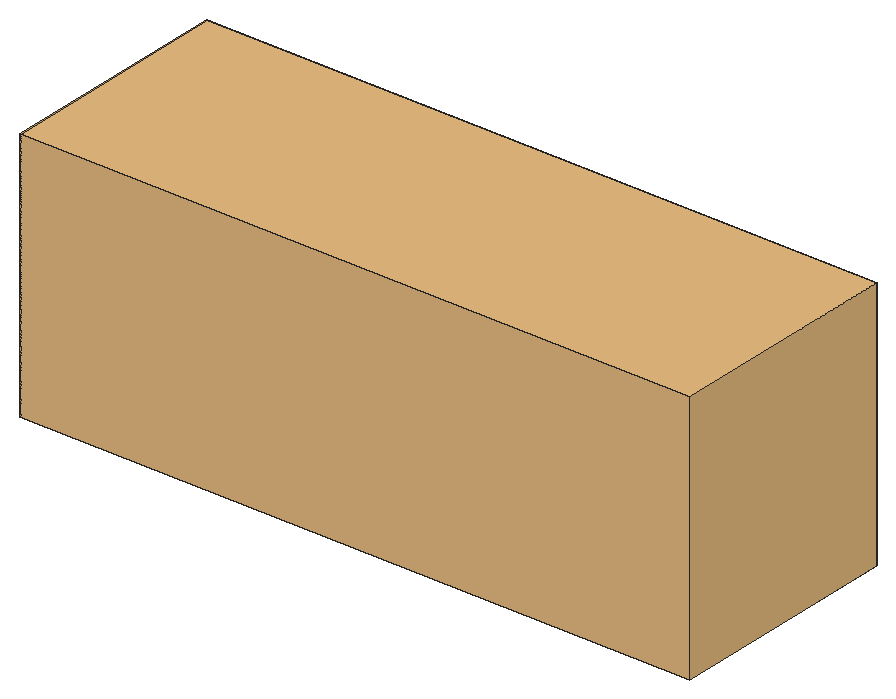
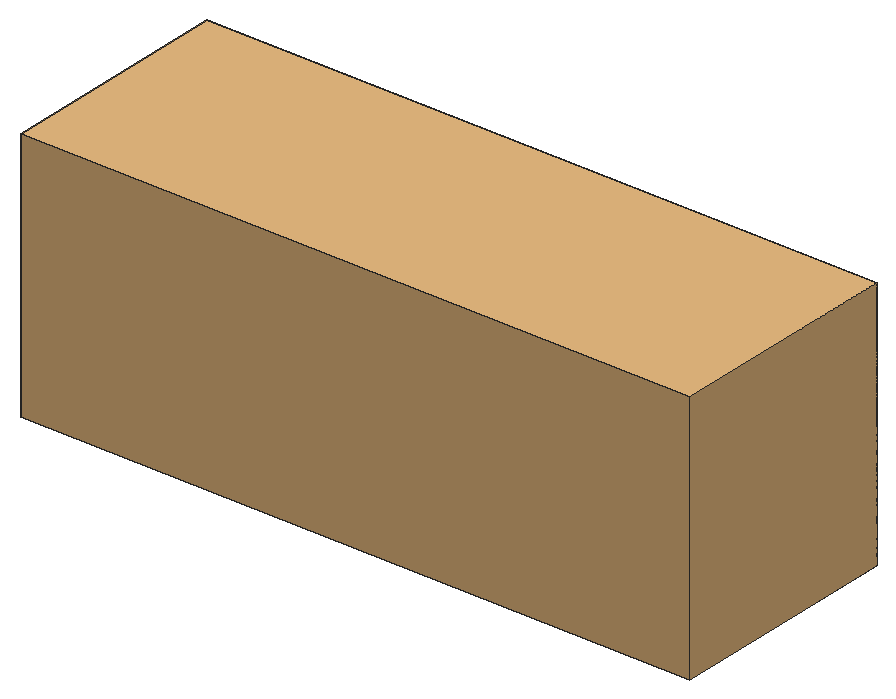
# SketchUp Ruby script. Lengths in inches.
U = 1.inch
M = Sketchup.active_model
def pt(a) = Geom::Point3d.new(a.map { |v| v * U })
def face(e, loops, mat)
  f = e.add_face(loops[0].map { |a| pt(a) })
  loops[1..].each { |l| e.add_face(l.map { |a| pt(a) }).erase! }
  f.material = f.back_material = mat if mat
  f
end
# faces: each face lists its corners as indices into pts; further lists are holes
def faces(e, pts, list, mat = nil) = list.each { |f| face(e, (f[0].is_a?(Array) ? f : [f]).map { |l| l.map { |i| pts[i] } }, mat) }
# xy, xz, yz: faces in a plane at the given z, y or x. An outline is a flat list of corners, or four numbers for a rectangle; further outlines are holes
def ring(l) = l.size == 4 ? [[l[0], l[1]], [l[2], l[1]], [l[2], l[3]], [l[0], l[3]]] : l.each_slice(2).to_a
def flat(e, list, mat, &to3) = list.each { |f| face(e, (f[0].is_a?(Array) ? f : [f]).map { |l| ring(l).map { |u, v| to3.(u, v) } }, mat) }
def xy(e, z, list, mat = nil) = flat(e, list, mat) { |x, y| [x, y, z] }
def xz(e, y, list, mat = nil) = flat(e, list, mat) { |x, z| [x, y, z] }
def yz(e, x, list, mat = nil) = flat(e, list, mat) { |y, z| [x, y, z] }
def lines(e, pts, list) = list.each { |a, b| e.add_line(pt(pts[a]), pt(pts[b])) }
# prism: a flat outline (further loops are holes) pulled along v
def prism(e, loops, v, mat = nil)
  f = face(e, loops, mat); d = Geom::Vector3d.new(v.map { |x| x * U })
  f.pushpull(f.normal.samedirection?(d) ? d.length : -d.length)
end
def box(e, o, s, mat = nil) = prism(e, [[o, [o[0] + s[0], o[1], o[2]], [o[0] + s[0], o[1] + s[1], o[2]], [o[0], o[1] + s[1], o[2]]]], [0, 0, s[2]], mat)
def at(x, y, z, deg = 0) = Geom::Transformation.translation(pt([x, y, z])) * Geom::Transformation.rotation(ORIGIN, Z_AXIS, deg.degrees)
def axes(o, x, y, z) = Geom::Transformation.new([*x, 0, *y, 0, *z, 0, *pt(o).to_a, 1])
def part(name) = M.definitions.add(name)
# library, detail: a bought-in or finely detailed component or shape, given as its bounding box
def library(name, o, s) = part(name).tap { |d| box(d.entities, o, s) }
def detail(e, o, s) = box(e.add_group.entities, o, s)
def put(e, d, t, mat = nil) = e.add_instance(d, t).tap { |i| i.material = mat if mat }
def group(e, t, mat = nil) = e.add_group.tap { |g| g.transformation = t; g.material = mat if mat }.entities
root = M.entities
M.materials.add("[Quartz Light Grey]").color = [251, 251, 252]
c1 = library("Group\#6",[0,-12,-12],[396,138,150])
xy(root,129,[[199.84,153,199.76,153.01,199.6875,153.02,199.61,153.03,199.45,153.05,199.375,153.07,199.3,153.08,199.22,153.1,199.15,153.125,199.07,153.15,199,153.17,198.92,153.2,198.71,153.29,198.64,153.33,198.57,153.36,198.43,153.44,198.37,153.48,198.3,153.53,198.24,153.57,198.17,153.62,197.93,153.82,197.88,153.88,197.82,153.93,197.62,154.17,197.57,154.24,197.53,154.3,197.48,154.37,197.44,154.43,197.36,154.57,197.33,154.64,197.29,154.71,197.2,154.92,197.17,155,197.15,155.07,197.125,155.15,197.1,155.22,197.08,155.3,197.07,155.375,197.05,155.45,197.03,155.61,197.02,155.6875,197.01,155.76,197,155.84,197,156.16,197.01,156.24,197.02,156.3125,197.03,156.39,197.05,156.55,197.07,156.625,197.08,156.7,197.1,156.78,197.125,156.85,197.15,156.93,197.17,157,197.2,157.08,197.29,157.29,197.33,157.36,197.36,157.43,197.44,157.57,197.48,157.63,197.53,157.7,197.57,157.76,197.62,157.83,197.82,158.07,197.88,158.12,197.93,158.18,198.17,158.38,198.24,158.43,198.3,158.47,198.37,158.52,198.43,158.56,198.57,158.64,198.64,158.67,198.71,158.71,198.92,158.8,199,158.83,199.07,158.85,199.15,158.875,199.22,158.9,199.3,158.92,199.375,158.93,199.45,158.95,199.61,158.97,199.6875,158.98,199.76,158.99,199.84,159,200.16,159,200.24,158.99,200.3125,158.98,200.39,158.97,200.55,158.95,200.625,158.93,200.7,158.92,200.78,158.9,200.85,158.875,200.93,158.85,201,158.83,201.08,158.8,201.29,158.71,201.36,158.67,201.43,158.64,201.57,158.56,201.63,158.52,201.7,158.47,201.76,158.43,201.83,158.38,202.07,158.18,202.12,158.12,202.18,158.07,202.38,157.83,202.43,157.76,202.47,157.7,202.52,157.63,202.56,157.57,202.64,157.43,202.67,157.36,202.71,157.29,202.8,157.08,202.83,157,202.85,156.93,202.875,156.85,202.9,156.78,202.92,156.7,202.93,156.625,202.95,156.55,202.97,156.39,202.98,156.3125,202.99,156.24,203,156.16,203,155.84,202.99,155.76,202.98,155.6875,202.97,155.61,202.95,155.45,202.93,155.375,202.92,155.3,202.9,155.22,202.875,155.15,202.85,155.07,202.83,155,202.8,154.92,202.71,154.71,202.67,154.64,202.64,154.57,202.56,154.43,202.52,154.37,202.47,154.3,202.43,154.24,202.38,154.17,202.18,153.93,202.12,153.88,202.07,153.82,201.83,153.62,201.76,153.57,201.7,153.53,201.63,153.48,201.57,153.44,201.43,153.36,201.36,153.33,201.29,153.29,201.08,153.2,201,153.17,200.93,153.15,200.85,153.125,200.78,153.1,200.7,153.08,200.625,153.07,200.55,153.05,200.39,153.03,200.3125,153.02,200.24,153.01,200.16,153]])
xz(root,96,[[48,128,426,132]])
xz(root,153,[[199.84,128,199.92,129],[199.92,128,200,129],[200,128,200.08,129],[200.08,128,200.16,129]])
xz(root,159,[[199.84,128,199.92,129],[199.92,128,200,129],[200,128,200.08,129],[200.08,128,200.16,129]])
yz(root,203,[[155.84,128,155.92,129],[155.92,128,156,129],[156,128,156.08,129],[156.08,128,156.16,129]])
yz(root,277,[[155.84,128,155.92,129],[155.92,128,156,129],[156,128,156.08,129],[156.08,128,156.16,129]])
p = [[199.53,153.04,128],[199.45,153.05,128],[199.45,153.05,129],[199.53,153.04,129],[199.61,153.03,128],[199.61,153.03,129],
  [199.6875,153.02,128],[199.6875,153.02,129],[199.76,153.01,128],[199.76,153.01,129],[199.84,153,128],[199.84,153,129],
  [200.24,153.01,128],[200.16,153,128],[200.16,153,129],[200.24,153.01,129],[200.3125,153.02,128],[200.3125,153.02,129],
  [200.39,153.03,128],[200.39,153.03,129],[200.47,153.04,128],[200.47,153.04,129],[200.55,153.05,128],[200.55,153.05,129],
  [279.53,153.04,128],[279.45,153.05,128],[279.45,153.05,129],[279.53,153.04,129],[279.61,153.03,128],[279.61,153.03,129],
  [279.6875,153.02,128],[279.6875,153.02,129],[279.76,153.01,128],[279.76,153.01,129],[199.07,153.15,128],[199,153.17,128],
  [199,153.17,129],[199.07,153.15,129],[199.15,153.125,128],[199.15,153.125,129],[199.22,153.1,128],[199.22,153.1,129],
  [199.3,153.08,128],[199.3,153.08,129],[199.375,153.07,128],[199.375,153.07,129],[200.625,153.07,128],[200.625,153.07,129],
  [200.7,153.08,128],[200.7,153.08,129],[200.78,153.1,128],[200.78,153.1,129],[200.85,153.125,128],[200.85,153.125,129],
  [200.93,153.15,128],[200.93,153.15,129],[201,153.17,128],[201,153.17,129],[279.07,153.15,128],[279,153.17,128],
  [279,153.17,129],[279.07,153.15,129],[279.15,153.125,128],[279.15,153.125,129],[279.22,153.1,128],[279.22,153.1,129],
  [279.3,153.08,128],[279.3,153.08,129],[279.375,153.07,128],[279.375,153.07,129],[198.85,153.23,128],[198.78,153.26,128],
  [198.78,153.26,129],[198.85,153.23,129],[198.92,153.2,128],[198.92,153.2,129],[201.08,153.2,128],[201.08,153.2,129],
  [201.15,153.23,128],[201.15,153.23,129],[201.22,153.26,128],[201.22,153.26,129],[278.85,153.23,128],[278.78,153.26,128],
  [278.78,153.26,129],[278.85,153.23,129],[278.92,153.2,128],[278.92,153.2,129],[198.64,153.33,128],[198.57,153.36,128],
  [198.57,153.36,129],[198.64,153.33,129],[198.71,153.29,128],[198.71,153.29,129],[201.29,153.29,128],[201.29,153.29,129],
  [201.36,153.33,128],[201.36,153.33,129],[201.43,153.36,128],[201.43,153.36,129],[278.64,153.33,128],[278.57,153.36,128],
  [278.57,153.36,129],[278.64,153.33,129],[278.71,153.29,128],[278.71,153.29,129],[198.43,153.44,128],[198.37,153.48,128],
  [198.37,153.48,129],[198.43,153.44,129],[198.5,153.4,128],[198.5,153.4,129],[201.5,153.4,128],[201.5,153.4,129],
  [201.57,153.44,128],[201.57,153.44,129],[201.63,153.48,128],[201.63,153.48,129],[278.43,153.44,128],[278.37,153.48,128],
  [278.37,153.48,129],[278.43,153.44,129],[278.5,153.4,128],[278.5,153.4,129],[198.3,153.53,128],[198.24,153.57,128],
  [198.24,153.57,129],[198.3,153.53,129],[201.7,153.53,128],[201.7,153.53,129],[201.76,153.57,128],[201.76,153.57,129],
  [278.3,153.53,128],[278.24,153.57,128],[278.24,153.57,129],[278.3,153.53,129],[198.17,153.62,128],[198.11,153.67,128],
  [198.11,153.67,129],[198.17,153.62,129],[201.83,153.62,128],[201.83,153.62,129],[201.89,153.67,128],[201.89,153.67,129],
  [278.17,153.62,128],[278.11,153.67,128],[278.11,153.67,129],[278.17,153.62,129],[198.05,153.72,128],[197.99,153.77,128],
  [197.99,153.77,129],[198.05,153.72,129],[201.95,153.72,128],[201.95,153.72,129],[202.01,153.77,128],[202.01,153.77,129],
  [278.05,153.72,128],[277.99,153.77,128],[277.99,153.77,129],[278.05,153.72,129],[197.93,153.82,128],[197.88,153.88,128],
  [197.88,153.88,129],[197.93,153.82,129],[202.07,153.82,128],[202.07,153.82,129],[202.12,153.88,128],[202.12,153.88,129],
  [277.93,153.82,128],[277.88,153.88,128],[277.88,153.88,129],[277.93,153.82,129],[197.82,153.93,128],[197.77,153.99,128],
  [197.77,153.99,129],[197.82,153.93,129],[202.18,153.93,128],[202.18,153.93,129],[202.23,153.99,128],[202.23,153.99,129],
  [277.82,153.93,128],[277.77,153.99,128],[277.77,153.99,129],[277.82,153.93,129],[202.28,154.05,128],[202.28,154.05,129],
  [277.72,154.05,128],[277.72,154.05,129],[202.33,154.11,128],[202.33,154.11,129],[202.38,154.17,128],[202.38,154.17,129],
  [277.67,154.11,128],[277.62,154.17,128],[277.62,154.17,129],[277.67,154.11,129],[202.43,154.24,128],[202.43,154.24,129],
  [202.47,154.3,128],[202.47,154.3,129],[277.57,154.24,128],[277.53,154.3,128],[277.53,154.3,129],[277.57,154.24,129],
  [202.52,154.37,128],[202.52,154.37,129],[277.48,154.37,128],[277.48,154.37,129],[202.56,154.43,128],[202.56,154.43,129],
  [202.6,154.5,128],[202.6,154.5,129],[277.44,154.43,128],[277.4,154.5,128],[277.4,154.5,129],[277.44,154.43,129],
  [202.64,154.57,128],[202.64,154.57,129],[277.36,154.57,128],[277.36,154.57,129],[202.67,154.64,128],[202.67,154.64,129],
  [202.71,154.71,128],[202.71,154.71,129],[277.33,154.64,128],[277.29,154.71,128],[277.29,154.71,129],[277.33,154.64,129],
  [202.74,154.78,128],[202.74,154.78,129],[277.26,154.78,128],[277.26,154.78,129],[202.77,154.85,128],[202.77,154.85,129],
  [277.23,154.85,128],[277.23,154.85,129],[202.8,154.92,128],[202.8,154.92,129],[202.83,155,128],[202.83,155,129],
  [277.2,154.92,128],[277.17,155,128],[277.17,155,129],[277.2,154.92,129],[202.85,155.07,128],[202.85,155.07,129],
  [277.15,155.07,128],[277.15,155.07,129],[202.875,155.15,128],[202.875,155.15,129],[202.9,155.22,128],[202.9,155.22,129],
  [277.125,155.15,128],[277.1,155.22,128],[277.1,155.22,129],[277.125,155.15,129],[202.92,155.3,128],[202.92,155.3,129],
  [277.08,155.3,128],[277.08,155.3,129],[202.93,155.375,128],[202.93,155.375,129],[277.07,155.375,128],[277.07,155.375,129],
  [202.95,155.45,128],[202.95,155.45,129],[277.05,155.45,128],[277.05,155.45,129],[202.96,155.53,128],[202.96,155.53,129],
  [202.97,155.61,128],[202.97,155.61,129],[277.04,155.53,128],[277.03,155.61,128],[277.03,155.61,129],[277.04,155.53,129],
  [202.98,155.6875,128],[202.98,155.6875,129],[277.02,155.6875,128],[277.02,155.6875,129],[202.99,155.76,128],[202.99,155.76,129],
  [277.01,155.76,128],[277.01,155.76,129],[203,155.84,128],[203,155.84,129],[277,155.84,128],[277,155.84,129],
  [202.98,156.3125,128],[202.99,156.24,128],[202.99,156.24,129],[202.98,156.3125,129],[203,156.16,128],[203,156.16,129],
  [277,156.16,128],[277.01,156.24,128],[277.01,156.24,129],[277,156.16,129],[277.02,156.3125,128],[277.02,156.3125,129],
  [202.97,156.39,128],[202.97,156.39,129],[277.03,156.39,128],[277.03,156.39,129],[202.96,156.47,128],[202.96,156.47,129],
  [277.04,156.47,128],[277.04,156.47,129],[202.93,156.625,128],[202.95,156.55,128],[202.95,156.55,129],[202.93,156.625,129],
  [277.05,156.55,128],[277.05,156.55,129],[277.07,156.625,128],[277.07,156.625,129],[202.92,156.7,128],[202.92,156.7,129],
  [277.08,156.7,128],[277.08,156.7,129],[202.9,156.78,128],[202.9,156.78,129],[277.1,156.78,128],[277.1,156.78,129],
  [202.875,156.85,128],[202.875,156.85,129],[277.125,156.85,128],[277.125,156.85,129],[202.83,157,128],[202.85,156.93,128],
  [202.85,156.93,129],[202.83,157,129],[277.15,156.93,128],[277.15,156.93,129],[277.17,157,128],[277.17,157,129],
  [202.8,157.08,128],[202.8,157.08,129],[277.2,157.08,128],[277.2,157.08,129],[202.74,157.22,128],[202.77,157.15,128],
  [202.77,157.15,129],[202.74,157.22,129],[277.23,157.15,128],[277.23,157.15,129],[277.26,157.22,128],[277.26,157.22,129],
  [202.71,157.29,128],[202.71,157.29,129],[277.29,157.29,128],[277.29,157.29,129],[202.67,157.36,128],[202.67,157.36,129],
  [277.33,157.36,128],[277.33,157.36,129],[202.6,157.5,128],[202.64,157.43,128],[202.64,157.43,129],[202.6,157.5,129],
  [277.36,157.43,128],[277.36,157.43,129],[277.4,157.5,128],[277.4,157.5,129],[202.56,157.57,128],[202.56,157.57,129],
  [277.44,157.57,128],[277.44,157.57,129],[202.47,157.7,128],[202.52,157.63,128],[202.52,157.63,129],[202.47,157.7,129],
  [277.48,157.63,128],[277.48,157.63,129],[277.53,157.7,128],[277.53,157.7,129],[202.43,157.76,128],[202.43,157.76,129],
  [277.57,157.76,128],[277.57,157.76,129],[202.33,157.89,128],[202.38,157.83,128],[202.38,157.83,129],[202.33,157.89,129],
  [277.62,157.83,128],[277.62,157.83,129],[277.67,157.89,128],[277.67,157.89,129],[202.23,158.01,128],[202.28,157.95,128],
  [202.28,157.95,129],[202.23,158.01,129],[277.72,157.95,128],[277.72,157.95,129],[277.77,158.01,128],[277.77,158.01,129],
  [202.18,158.07,128],[202.18,158.07,129],[277.82,158.07,128],[277.82,158.07,129],[197.82,158.07,128],[197.88,158.12,128],
  [197.88,158.12,129],[197.82,158.07,129],[197.93,158.18,128],[197.93,158.18,129],[202.07,158.18,128],[202.12,158.12,128],
  [202.12,158.12,129],[202.07,158.18,129],[277.88,158.12,128],[277.88,158.12,129],[277.93,158.18,128],[277.93,158.18,129],
  [197.99,158.23,128],[197.99,158.23,129],[198.05,158.28,128],[198.05,158.28,129],[201.95,158.28,128],[202.01,158.23,128],
  [202.01,158.23,129],[201.95,158.28,129],[277.99,158.23,128],[277.99,158.23,129],[278.05,158.28,128],[278.05,158.28,129],
  [198.11,158.33,128],[198.11,158.33,129],[198.17,158.38,128],[198.17,158.38,129],[201.83,158.38,128],[201.89,158.33,128],
  [201.89,158.33,129],[201.83,158.38,129],[278.11,158.33,128],[278.11,158.33,129],[278.17,158.38,128],[278.17,158.38,129],
  [198.24,158.43,128],[198.24,158.43,129],[198.3,158.47,128],[198.3,158.47,129],[201.7,158.47,128],[201.76,158.43,128],
  [201.76,158.43,129],[201.7,158.47,129],[278.24,158.43,128],[278.24,158.43,129],[278.3,158.47,128],[278.3,158.47,129],
  [198.37,158.52,128],[198.37,158.52,129],[198.43,158.56,128],[198.43,158.56,129],[201.57,158.56,128],[201.63,158.52,128],
  [201.63,158.52,129],[201.57,158.56,129],[278.37,158.52,128],[278.37,158.52,129],[278.43,158.56,128],[278.43,158.56,129],
  [198.5,158.6,128],[198.5,158.6,129],[198.57,158.64,128],[198.57,158.64,129],[198.64,158.67,128],[198.64,158.67,129],
  [201.36,158.67,128],[201.43,158.64,128],[201.43,158.64,129],[201.36,158.67,129],[201.5,158.6,128],[201.5,158.6,129],
  [278.5,158.6,128],[278.5,158.6,129],[278.57,158.64,128],[278.57,158.64,129],[278.64,158.67,128],[278.64,158.67,129],
  [198.71,158.71,128],[198.71,158.71,129],[198.78,158.74,128],[198.78,158.74,129],[198.85,158.77,128],[198.85,158.77,129],
  [201.15,158.77,128],[201.22,158.74,128],[201.22,158.74,129],[201.15,158.77,129],[201.29,158.71,128],[201.29,158.71,129],
  [278.71,158.71,128],[278.71,158.71,129],[278.78,158.74,128],[278.78,158.74,129],[278.85,158.77,128],[278.85,158.77,129],
  [198.92,158.8,128],[198.92,158.8,129],[199,158.83,128],[199,158.83,129],[199.07,158.85,128],[199.07,158.85,129],
  [200.93,158.85,128],[201,158.83,128],[201,158.83,129],[200.93,158.85,129],[201.08,158.8,128],[201.08,158.8,129],
  [278.92,158.8,128],[278.92,158.8,129],[279,158.83,128],[279,158.83,129],[279.07,158.85,128],[279.07,158.85,129],
  [199.15,158.875,128],[199.15,158.875,129],[199.22,158.9,128],[199.22,158.9,129],[199.3,158.92,128],[199.3,158.92,129],
  [199.375,158.93,128],[199.375,158.93,129],[199.45,158.95,128],[199.45,158.95,129],[199.53,158.96,128],[199.53,158.96,129],
  [200.47,158.96,128],[200.55,158.95,128],[200.55,158.95,129],[200.47,158.96,129],[200.625,158.93,128],[200.625,158.93,129],
  [200.7,158.92,128],[200.7,158.92,129],[200.78,158.9,128],[200.78,158.9,129],[200.85,158.875,128],[200.85,158.875,129],
  [279.15,158.875,128],[279.15,158.875,129],[279.22,158.9,128],[279.22,158.9,129],[279.3,158.92,128],[279.3,158.92,129],
  [279.375,158.93,128],[279.375,158.93,129],[279.45,158.95,128],[279.45,158.95,129],[279.53,158.96,128],[279.53,158.96,129],
  [199.61,158.97,128],[199.61,158.97,129],[199.6875,158.98,128],[199.6875,158.98,129],[199.76,158.99,128],[199.76,158.99,129],
  [199.84,159,128],[199.84,159,129],[200.16,159,128],[200.24,158.99,128],[200.24,158.99,129],[200.16,159,129],
  [200.3125,158.98,128],[200.3125,158.98,129],[200.39,158.97,128],[200.39,158.97,129],[279.61,158.97,128],[279.61,158.97,129],
  [279.6875,158.98,128],[279.6875,158.98,129]]
faces(root,p,[[0,1,2,3],[4,0,3,5],[6,4,5,7],[8,6,7,9],[10,8,9,11],[12,13,14,15],[16,12,15,17],[18,16,17,19],
  [20,18,19,21],[22,20,21,23],[24,25,26,27],[28,24,27,29],[30,28,29,31],[32,30,31,33],[34,35,36,37],[38,34,37,39],
  [40,38,39,41],[42,40,41,43],[44,42,43,45],[1,44,45,2],[46,22,23,47],[48,46,47,49],[50,48,49,51],[52,50,51,53],
  [54,52,53,55],[56,54,55,57],[58,59,60,61],[62,58,61,63],[64,62,63,65],[66,64,65,67],[68,66,67,69],[25,68,69,26],
  [70,71,72,73],[74,70,73,75],[35,74,75,36],[76,56,57,77],[78,76,77,79],[80,78,79,81],[82,83,84,85],[86,82,85,87],
  [59,86,87,60],[88,89,90,91],[92,88,91,93],[71,92,93,72],[94,80,81,95],[96,94,95,97],[98,96,97,99],[100,101,102,103],
  [104,100,103,105],[83,104,105,84],[106,107,108,109],[110,106,109,111],[89,110,111,90],[112,98,99,113],[114,112,113,115],[116,114,115,117],
  [118,119,120,121],[122,118,121,123],[101,122,123,102],[124,125,126,127],[107,124,127,108],[128,116,117,129],[130,128,129,131],[132,133,134,135],
  [119,132,135,120],[136,137,138,139],[125,136,139,126],[140,130,131,141],[142,140,141,143],[144,145,146,147],[133,144,147,134],[148,149,150,151],
  [137,148,151,138],[152,142,143,153],[154,152,153,155],[156,157,158,159],[145,156,159,146],[160,161,162,163],[149,160,163,150],[164,154,155,165],
  [166,164,165,167],[168,169,170,171],[157,168,171,158],[172,173,174,175],[161,172,175,162],[176,166,167,177],[178,176,177,179],[180,181,182,183],
  [169,180,183,170],[184,178,179,185],[181,186,187,182],[188,184,185,189],[190,188,189,191],[192,193,194,195],[186,192,195,187],[196,190,191,197],
  [198,196,197,199],[200,201,202,203],[193,200,203,194],[204,198,199,205],[201,206,207,202],[208,204,205,209],[210,208,209,211],[212,213,214,215],
  [206,212,215,207],[216,210,211,217],[213,218,219,214],[220,216,217,221],[222,220,221,223],[224,225,226,227],[218,224,227,219],[228,222,223,229],
  [225,230,231,226],[232,228,229,233],[230,234,235,231],[236,232,233,237],[238,236,237,239],[240,241,242,243],[234,240,243,235],[244,238,239,245],
  [241,246,247,242],[248,244,245,249],[250,248,249,251],[252,253,254,255],[246,252,255,247],[256,250,251,257],[253,258,259,254],[260,256,257,261],
  [258,262,263,259],[264,260,261,265],[262,266,267,263],[268,264,265,269],[270,268,269,271],[272,273,274,275],[266,272,275,267],[276,270,271,277],
  [273,278,279,274],[280,276,277,281],[278,282,283,279],[284,280,281,285],[282,286,287,283],[288,289,290,291],[289,292,293,290],[294,295,296,297],
  [295,298,299,296],[300,288,291,301],[298,302,303,299],[304,300,301,305],[302,306,307,303],[308,309,310,311],[309,304,305,310],[306,312,313,307],
  [312,314,315,313],[316,308,311,317],[314,318,319,315],[320,316,317,321],[318,322,323,319],[324,320,321,325],[322,326,327,323],[328,329,330,331],
  [329,324,325,330],[326,332,333,327],[332,334,335,333],[336,328,331,337],[334,338,339,335],[340,341,342,343],[341,336,337,342],[338,344,345,339],
  [344,346,347,345],[348,340,343,349],[346,350,351,347],[352,348,349,353],[350,354,355,351],[356,357,358,359],[357,352,353,358],[354,360,361,355],
  [360,362,363,361],[364,356,359,365],[362,366,367,363],[368,369,370,371],[369,364,365,370],[366,372,373,367],[372,374,375,373],[376,368,371,377],
  [374,378,379,375],[380,381,382,383],[381,376,377,382],[378,384,385,379],[384,386,387,385],[388,389,390,391],[389,380,383,390],[386,392,393,387],
  [392,394,395,393],[396,388,391,397],[394,398,399,395],[400,401,402,403],[401,404,405,402],[406,407,408,409],[407,396,397,408],[398,410,411,399],
  [410,412,413,411],[404,414,415,405],[414,416,417,415],[418,419,420,421],[419,406,409,420],[412,422,423,413],[422,424,425,423],[416,426,427,417],
  [426,428,429,427],[430,431,432,433],[431,418,421,432],[424,434,435,425],[434,436,437,435],[428,438,439,429],[438,440,441,439],[442,443,444,445],
  [443,430,433,444],[436,446,447,437],[446,448,449,447],[440,450,451,441],[450,452,453,451],[454,455,456,457],[455,442,445,456],[448,458,459,449],
  [458,460,461,459],[452,462,463,453],[462,464,465,463],[464,466,467,465],[468,469,470,471],[469,472,473,470],[472,454,457,473],[460,474,475,461],
  [474,476,477,475],[476,478,479,477],[466,480,481,467],[480,482,483,481],[482,484,485,483],[486,487,488,489],[487,490,491,488],[490,468,471,491],
  [478,492,493,479],[492,494,495,493],[494,496,497,495],[484,498,499,485],[498,500,501,499],[500,502,503,501],[504,505,506,507],[505,508,509,506],
  [508,486,489,509],[496,510,511,497],[510,512,513,511],[512,514,515,513],[502,516,517,503],[516,518,519,517],[518,520,521,519],[520,522,523,521],
  [522,524,525,523],[524,526,527,525],[528,529,530,531],[529,532,533,530],[532,534,535,533],[534,536,537,535],[536,538,539,537],[538,504,507,539],
  [514,540,541,515],[540,542,543,541],[542,544,545,543],[544,546,547,545],[546,548,549,547],[548,550,551,549],[526,552,553,527],[552,554,555,553],
  [554,556,557,555],[556,558,559,557],[560,561,562,563],[561,564,565,562],[564,566,567,565],[566,528,531,567],[550,568,569,551],[568,570,571,569]])
put(root,c1,at(48,90,138),"[Quartz Light Grey]")
